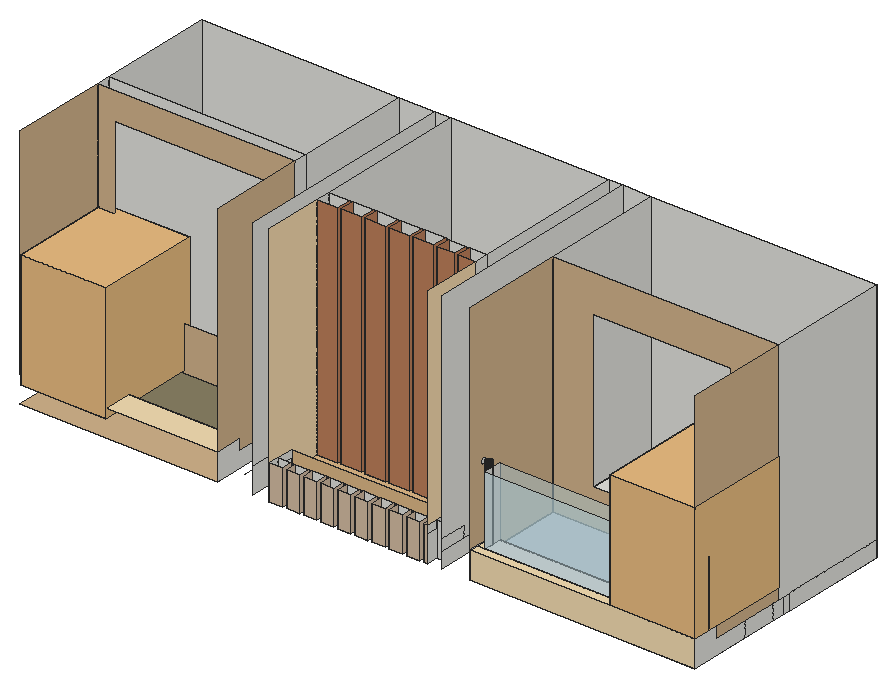
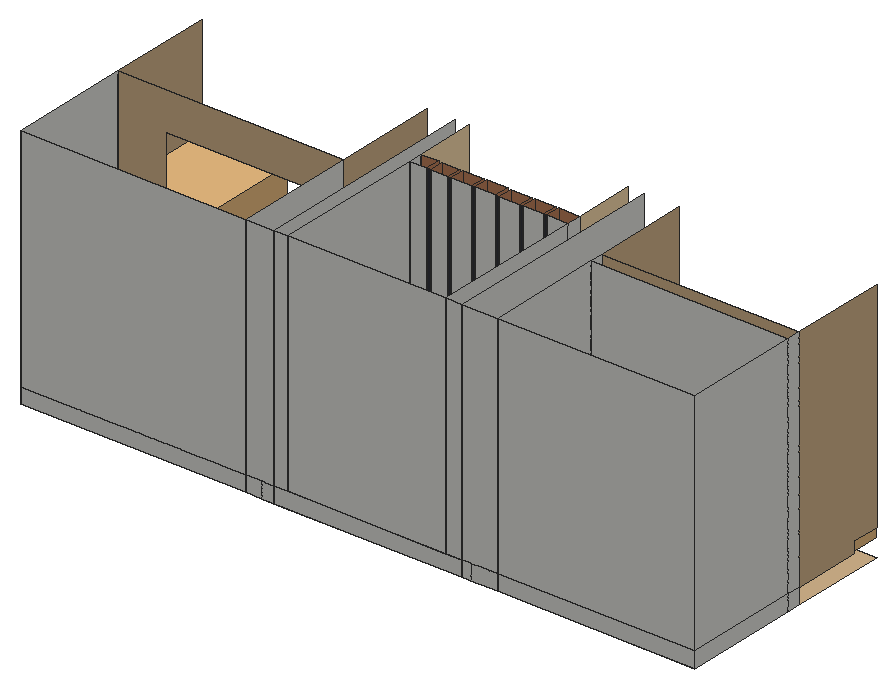
# SketchUp Ruby script. Lengths in inches.
U = 1.inch
M = Sketchup.active_model
def pt(a) = Geom::Point3d.new(a.map { |v| v * U })
def face(e, loops, mat)
  f = e.add_face(loops[0].map { |a| pt(a) })
  loops[1..].each { |l| e.add_face(l.map { |a| pt(a) }).erase! }
  f.material = f.back_material = mat if mat
  f
end
# faces: each face lists its corners as indices into pts; further lists are holes
def faces(e, pts, list, mat = nil) = list.each { |f| face(e, (f[0].is_a?(Array) ? f : [f]).map { |l| l.map { |i| pts[i] } }, mat) }
# xy, xz, yz: faces in a plane at the given z, y or x. An outline is a flat list of corners, or four numbers for a rectangle; further outlines are holes
def ring(l) = l.size == 4 ? [[l[0], l[1]], [l[2], l[1]], [l[2], l[3]], [l[0], l[3]]] : l.each_slice(2).to_a
def flat(e, list, mat, &to3) = list.each { |f| face(e, (f[0].is_a?(Array) ? f : [f]).map { |l| ring(l).map { |u, v| to3.(u, v) } }, mat) }
def xy(e, z, list, mat = nil) = flat(e, list, mat) { |x, y| [x, y, z] }
def xz(e, y, list, mat = nil) = flat(e, list, mat) { |x, z| [x, y, z] }
def yz(e, x, list, mat = nil) = flat(e, list, mat) { |y, z| [x, y, z] }
def lines(e, pts, list) = list.each { |a, b| e.add_line(pt(pts[a]), pt(pts[b])) }
# prism: a flat outline (further loops are holes) pulled along v
def prism(e, loops, v, mat = nil)
  f = face(e, loops, mat); d = Geom::Vector3d.new(v.map { |x| x * U })
  f.pushpull(f.normal.samedirection?(d) ? d.length : -d.length)
end
def box(e, o, s, mat = nil) = prism(e, [[o, [o[0] + s[0], o[1], o[2]], [o[0] + s[0], o[1] + s[1], o[2]], [o[0], o[1] + s[1], o[2]]]], [0, 0, s[2]], mat)
def at(x, y, z, deg = 0) = Geom::Transformation.translation(pt([x, y, z])) * Geom::Transformation.rotation(ORIGIN, Z_AXIS, deg.degrees)
def axes(o, x, y, z) = Geom::Transformation.new([*x, 0, *y, 0, *z, 0, *pt(o).to_a, 1])
def part(name) = M.definitions.add(name)
# library, detail: a bought-in or finely detailed component or shape, given as its bounding box
def library(name, o, s) = part(name).tap { |d| box(d.entities, o, s) }
def detail(e, o, s) = box(e.add_group.entities, o, s)
def put(e, d, t, mat = nil) = e.add_instance(d, t).tap { |i| i.material = mat if mat }
def group(e, t, mat = nil) = e.add_group.tap { |g| g.transformation = t; g.material = mat if mat }.entities
root = M.entities
M.materials.add("[0027_PeachPuff]").color = [255, 218, 185]
M.materials.add("[0034_Wheat]").color = [245, 222, 179]
M.materials.add("[0035_Tan]").color = [210, 180, 140]
M.materials.add("[0036_BurlyWood]1").color = [222, 184, 135]
M.materials.add("[Carpet Pattern Squares Multi]").color = [138, 129, 101]
M.materials.add("[Formica Beige]").color = [247, 219, 174]
M.materials.add("[Formica Laminate Dark]").color = [50, 53, 60]
M.materials.add("[Formica Laminate Light]").color = [213, 189, 164]
M.materials.add("[Marble Carrara Floor Tile]").color = [204, 208, 219]
M.materials.add("[Translucent Glass Safety]").color = [204, 235, 244]
M.materials["[Translucent Glass Safety]"].alpha = 0.5
M.materials.add("[Wood Veneer 02]").color = [190, 128, 91]
c1 = library("chau cay",[-24.34,-109.24,0],[56.46,62.58,79.69])
xy(root,1615.875,[[800.41,433.79,848.4,457.98],[856.53,433.79,904.52,457.98],[912.66,433.79,960.65,457.98],[968.78,433.79,1016.77,457.98],[1024.91,433.79,1072.9,457.98],
  [1081.03,433.79,1129.02,457.98],[1137.16,433.79,1185.15,457.98],[1192.22,433.79,1232.95,457.98],[1240.21,433.79,1272.8,457.98],[58.44,584.29,646.67,623.89],
  [646.67,584.29,752.97,623.89],[752.97,584.29,1313.62,623.89],[1313.62,584.29,1398.32,623.89],[58.44,623.89,646.67,971.67],[646.67,623.89,752.97,971.67],
  [752.97,623.89,1313.62,971.67],[1313.62,623.89,1398.32,971.67],[1398.32,647.48,2069.85,971.67]])
xy(root,1615.875,[[800.41,328.44,800.41,433.79,848.4,433.79,848.4,457.98,856.53,457.98,856.53,433.79,904.52,433.79,904.52,457.98,912.66,457.98,912.66,433.79,960.65,433.79,960.65,457.98,968.78,457.98,968.78,433.79,1016.77,433.79,1016.77,457.98,1024.91,457.98,1024.91,433.79,1072.9,433.79,1072.9,457.98,1081.03,457.98,1081.03,433.79,1129.02,433.79,1129.02,457.98,1137.16,457.98,1137.16,433.79,1185.15,433.79,1185.15,457.98,1192.22,457.98,1192.22,433.79,1232.95,433.79,1232.95,457.98,1240.21,457.98,1240.21,433.79,1272.8,433.79,1272.8,328.44]],"[0027_PeachPuff]")
xy(root,1615.875,[[58.44,295.82,646.67,584.29],[1398.32,295.82,2069.85,584.29],[1398.32,584.29,2069.85,623.89],[1398.32,623.89,2069.85,647.48]],"[0035_Tan]")
xy(root,1615.875,[[800.41,295.82,840.05,328.44],[851.53,295.82,891.17,328.44],[902.66,295.82,942.3,328.44],[953.78,295.82,993.42,328.44],[1004.91,295.82,1044.55,328.44],
  [1056.03,295.82,1095.67,328.44],[1107.16,295.82,1146.8,328.44],[1158.28,295.82,1197.92,328.44],[1209.41,295.82,1249.05,328.44],[1260.53,295.82,1272.8,328.44]],"[Formica Laminate Light]")
xy(root,1662.5625,[[752.97,378.54,800.41,971.67],[1272.8,378.54,1313.62,971.67],[800.41,474.79,862.92,517.1],[871.91,474.79,934.42,517.1],[943.41,474.79,1005.92,517.1],
  [1014.91,474.79,1077.42,517.1],[1086.41,474.79,1148.92,517.1],[1157.91,474.79,1210.375,517.1],[1220.42,474.79,1272.8,517.1],[800.41,517.1,1272.8,971.67],
  [58.44,584.29,646.67,623.89],[1398.32,606.67,2069.85,971.67],[58.44,623.89,646.67,971.67]])
xy(root,1662.5625,[[800.41,378.54,1272.8,378.54,1272.8,474.79,1220.42,474.79,1220.42,517.1,1210.375,517.1,1210.375,474.79,1157.91,474.79,1157.91,517.1,1148.92,517.1,1148.92,474.79,1086.41,474.79,1086.41,517.1,1077.42,517.1,1077.42,474.79,1014.91,474.79,1014.91,517.1,1005.92,517.1,1005.92,474.79,943.41,474.79,943.41,517.1,934.42,517.1,934.42,474.79,871.91,474.79,871.91,517.1,862.92,517.1,862.92,474.79,800.41,474.79]],"[0036_BurlyWood]1")
xy(root,1662.5625,[[58.44,378.54,646.67,584.29]],"[Carpet Pattern Squares Multi]")
xy(root,1662.5625,[[1398.32,378.54,2069.85,606.67]],"[Marble Carrara Floor Tile]")
xy(root,1695.75,[[1423.33,322.36,2046.06,378.54],[1413.02,338.97,1411.98,339.01,1410.95,339.17,1409.95,339.43,1408.97,339.8,1408.04,340.27,1407.17,340.83,1406.36,341.48,1405.62,342.21,1404.96,343.02,1404.39,343.89,1403.91,344.81,1403.53,345.78,1403.26,346.78,1403.09,347.81,1403.03,348.85,1403.08,349.89,1403.23,350.91,1403.5,351.92,1403.86,352.89,1404.33,353.82,1404.89,354.7,1405.54,355.51,1406.27,356.25,1407.08,356.91,1407.95,357.48,1408.87,357.96,1409.84,358.34,1410.84,358.61,1411.87,358.78,1412.91,358.84,1413.95,358.79,1414.97,358.64,1415.98,358.37,1416.95,358,1417.88,357.54,1418.76,356.98,1419.57,356.33,1420.3125,355.59,1420.97,354.79,1421.54,353.92,1422.02,353,1422.4,352.03,1422.67,351.02,1422.84,350,1422.9,348.96,1422.85,347.92,1422.7,346.89,1422.43,345.89,1422.07,344.91,1421.6,343.98,1421.04,343.11,1420.39,342.3,1419.66,341.56,1418.85,340.9,1417.98,340.33,1417.06,339.85,1416.09,339.47,1415.09,339.19,1414.06,339.03],[2056.33,338.97,2055.29,339.01,2054.27,339.17,2053.26,339.43,2052.29,339.8,2051.36,340.27,2050.48,340.83,2049.67,341.48,2048.93,342.21,2048.27,343.02,2047.7,343.89,2047.22,344.81,2046.84,345.78,2046.57,346.78,2046.4,347.81,2046.34,348.85,2046.39,349.89,2046.54,350.91,2046.81,351.92,2047.18,352.89,2047.64,353.82,2048.2,354.7,2048.85,355.51,2049.58,356.25,2050.39,356.91,2051.26,357.48,2052.18,357.96,2053.15,358.34,2054.15,358.61,2055.18,358.78,2056.22,358.84,2057.26,358.79,2058.29,358.64,2059.29,358.37,2060.27,358,2061.2,357.54,2062.07,356.98,2062.88,356.33,2063.625,355.59,2064.28,354.79,2064.85,353.92,2065.33,353,2065.71,352.03,2065.98,351.02,2066.15,350,2066.21,348.96,2066.17,347.92,2066.01,346.89,2065.75,345.89,2065.38,344.91,2064.91,343.98,2064.35,343.11,2063.7,342.3,2062.97,341.56,2062.16,340.9,2061.29,340.33,2060.37,339.85,2059.4,339.47,2058.4,339.19,2057.37,339.03]])
xy(root,1695.75,[[58.44,295.82,646.67,378.54],[1398.32,295.82,2069.85,322.36],[[1398.32,322.36,1423.33,378.54],[1413.02,338.97,1411.98,339.01,1410.95,339.17,1409.95,339.43,1408.97,339.8,1408.04,340.27,1407.17,340.83,1406.36,341.48,1405.62,342.21,1404.96,343.02,1404.39,343.89,1403.91,344.81,1403.53,345.78,1403.26,346.78,1403.09,347.81,1403.03,348.85,1403.08,349.89,1403.23,350.91,1403.5,351.92,1403.86,352.89,1404.33,353.82,1404.89,354.7,1405.54,355.51,1406.27,356.25,1407.08,356.91,1407.95,357.48,1408.87,357.96,1409.84,358.34,1410.84,358.61,1411.87,358.78,1412.91,358.84,1413.95,358.79,1414.97,358.64,1415.98,358.37,1416.95,358,1417.88,357.54,1418.76,356.98,1419.57,356.33,1420.3125,355.59,1420.97,354.79,1421.54,353.92,1422.02,353,1422.4,352.03,1422.67,351.02,1422.84,350,1422.9,348.96,1422.85,347.92,1422.7,346.89,1422.43,345.89,1422.07,344.91,1421.6,343.98,1421.04,343.11,1420.39,342.3,1419.66,341.56,1418.85,340.9,1417.98,340.33,1417.06,339.85,1416.09,339.47,1415.09,339.19,1414.06,339.03]],[[2046.06,322.36,2069.85,378.54],[2056.33,338.97,2055.29,339.01,2054.27,339.17,2053.26,339.43,2052.29,339.8,2051.36,340.27,2050.48,340.83,2049.67,341.48,2048.93,342.21,2048.27,343.02,2047.7,343.89,2047.22,344.81,2046.84,345.78,2046.57,346.78,2046.4,347.81,2046.34,348.85,2046.39,349.89,2046.54,350.91,2046.81,351.92,2047.18,352.89,2047.64,353.82,2048.2,354.7,2048.85,355.51,2049.58,356.25,2050.39,356.91,2051.26,357.48,2052.18,357.96,2053.15,358.34,2054.15,358.61,2055.18,358.78,2056.22,358.84,2057.26,358.79,2058.29,358.64,2059.29,358.37,2060.27,358,2061.2,357.54,2062.07,356.98,2062.88,356.33,2063.625,355.59,2064.28,354.79,2064.85,353.92,2065.33,353,2065.71,352.03,2065.98,351.02,2066.15,350,2066.21,348.96,2066.17,347.92,2066.01,346.89,2065.75,345.89,2065.38,344.91,2064.91,343.98,2064.35,343.11,2063.7,342.3,2062.97,341.56,2062.16,340.9,2061.29,340.33,2060.37,339.85,2059.4,339.47,2058.4,339.19,2057.37,339.03]]],"[0034_Wheat]")
xz(root,295.82,[[1398.32,1615.875,2069.85,1695.75]],"[0034_Wheat]")
xz(root,295.82,[[800.41,1615.875,840.05,1718.875],[851.53,1615.875,891.17,1718.875],[902.66,1615.875,942.3,1718.875],[953.78,1615.875,993.42,1718.875],[1004.91,1615.875,1044.55,1718.875],
  [1056.03,1615.875,1095.67,1718.875],[1107.16,1615.875,1146.8,1718.875],[1158.28,1615.875,1197.92,1718.875],[1209.41,1615.875,1249.05,1718.875],[1260.53,1615.875,1272.8,1718.875]],"[Formica Laminate Light]")
xz(root,322.36,[[1423.33,1695.75,2046.06,1901.1875]],"[Translucent Glass Safety]")
xz(root,328.44,[[800.41,1615.875,840.05,1718.875],[851.53,1615.875,891.17,1718.875],[902.66,1615.875,942.3,1718.875],[953.78,1615.875,993.42,1718.875],[1004.91,1615.875,1044.55,1718.875],
  [1056.03,1615.875,1095.67,1718.875],[1107.16,1615.875,1146.8,1718.875],[1158.28,1615.875,1197.92,1718.875],[1209.41,1615.875,1249.05,1718.875],[1260.53,1615.875,1272.8,1718.875],
  [1272.8,1615.875,1300.17,1718.875]])
xz(root,328.44,[[840.05,1615.875,851.53,1718.875],[891.17,1615.875,902.66,1718.875],[942.3,1615.875,953.78,1718.875],[993.42,1615.875,1004.91,1718.875],[1044.55,1615.875,1056.03,1718.875],
  [1095.67,1615.875,1107.16,1718.875],[1146.8,1615.875,1158.28,1718.875],[1197.92,1615.875,1209.41,1718.875],[1249.05,1615.875,1260.53,1718.875]],"[Formica Laminate Dark]")
xz(root,378.54,[[752.97,1662.5625,800.41,1695.75],[1272.8,1662.5625,1313.62,1695.75],[1398.32,1662.5625,2069.85,1695.75]])
xz(root,378.54,[[58.44,1662.5625,646.67,1695.75]],"[0034_Wheat]")
xz(root,378.54,[[800.41,1662.5625,1272.8,1718.875]],"[0036_BurlyWood]1")
xz(root,378.54,[[1423.33,1695.75,2046.06,1901.1875]],"[Translucent Glass Safety]")
xz(root,474.79,[[800.41,1662.5625,862.92,2344.3125],[871.91,1662.5625,934.42,2344.3125],[943.41,1662.5625,1005.92,2344.3125],[1014.91,1662.5625,1077.42,2344.3125],[1086.41,1662.5625,1148.92,2344.3125],
  [1157.91,1662.5625,1210.375,2344.3125],[1220.42,1662.5625,1272.8,2344.3125]],"[Wood Veneer 02]")
xz(root,517.1,[[800.41,1662.5625,862.92,2344.3125],[871.91,1662.5625,934.42,2344.3125],[943.41,1662.5625,1005.92,2344.3125],[1014.91,1662.5625,1077.42,2344.3125],[1086.41,1662.5625,1148.92,2344.3125],
  [1157.91,1662.5625,1210.375,2344.3125],[1220.42,1662.5625,1272.8,2344.3125]])
xz(root,517.1,[[862.92,1662.5625,871.91,2344.3125],[934.42,1662.5625,943.41,2344.3125],[1005.92,1662.5625,1014.91,2344.3125],[1077.42,1662.5625,1086.41,2344.3125],[1148.92,1662.5625,1157.91,2344.3125],
  [1210.375,1662.5625,1220.42,2344.3125]],"[Formica Laminate Dark]")
xz(root,584.29,[[[58.44,1662.5625,646.67,2344.3125],[108.51,1794.2,576.32,2262.01]]],"[0035_Tan]")
xz(root,606.67,[[[1398.32,1662.5625,2069.85,2344.3125],[1516.53,1770.73,1927.28,2231.42]]],"[0035_Tan]")
xz(root,623.89,[[58.44,1662.5625,646.67,2344.3125]])
xz(root,971.67,[[58.44,1615.875,646.67,1662.5625],[646.67,1615.875,726.78,1662.5625],[726.78,1615.875,752.97,1662.5625],[752.97,1615.875,1313.62,1662.5625],[1313.62,1615.875,1351.23,1662.5625],
  [1351.23,1615.875,1398.32,1662.5625],[1398.32,1615.875,2069.85,1662.5625],[58.44,1662.5625,646.67,2344.3125],[646.67,1662.5625,752.97,2344.3125],[752.97,1662.5625,800.41,2344.3125],
  [800.41,1662.5625,1272.8,2344.3125],[1272.8,1662.5625,1313.62,2344.3125],[1313.62,1662.5625,1398.32,2344.3125],[1398.32,1662.5625,2069.85,2344.3125]])
yz(root,58.44,[[584.29,1615.875,623.89,1662.5625],[623.89,1615.875,971.67,1662.5625],[584.29,1662.5625,623.89,2344.3125],[623.89,1662.5625,971.67,2344.3125]])
yz(root,58.44,[[378.54,1662.5625,584.29,1662.5625,584.29,2344.3125,295.82,2344.3125,295.82,1695.75,378.54,1695.75]],"[0035_Tan]")
yz(root,646.67,[[295.82,1615.875,295.82,1695.75,378.54,1695.75,378.54,1662.5625,971.67,1662.5625,971.67,1615.875],[584.29,1662.5625,623.89,2344.3125],[623.89,1662.5625,971.67,2344.3125]])
yz(root,646.67,[[378.54,1662.5625,378.54,1695.75,295.82,1695.75,295.82,2344.3125,584.29,2344.3125,584.29,1662.5625]],"[0035_Tan]")
yz(root,752.97,[[295.82,1615.875,295.82,1695.75,378.54,1695.75,378.54,1662.5625,971.67,1662.5625,971.67,1615.875],[378.54,1662.5625,378.54,1695.75,295.82,1695.75,295.82,2344.3125,971.67,2344.3125,971.67,1662.5625]])
yz(root,800.41,[[295.82,1615.875,328.44,1695.75],[474.79,1662.5625,517.1,2344.3125],[517.1,1662.5625,971.67,2344.3125],[295.82,1695.75,328.44,1718.875],[328.44,1695.75,378.54,1718.875]])
yz(root,800.41,[[378.54,1662.5625,474.79,1662.5625,474.79,2344.3125,295.82,2344.3125,295.82,1718.875,378.54,1718.875]],"[Formica Beige]")
yz(root,840.05,[[295.82,1615.875,328.44,1718.875]],"[Formica Laminate Light]")
yz(root,851.53,[[295.82,1615.875,328.44,1695.75],[295.82,1695.75,328.44,1718.875]],"[Formica Laminate Light]")
yz(root,862.92,[[474.79,1662.5625,517.1,2344.3125]],"[Wood Veneer 02]")
yz(root,871.91,[[474.79,1662.5625,517.1,2344.3125]],"[Wood Veneer 02]")
yz(root,891.17,[[295.82,1615.875,328.44,1718.875]],"[Formica Laminate Light]")
yz(root,902.66,[[295.82,1615.875,328.44,1695.75],[295.82,1695.75,328.44,1718.875]],"[Formica Laminate Light]")
yz(root,934.42,[[474.79,1662.5625,517.1,2344.3125]],"[Wood Veneer 02]")
yz(root,942.3,[[295.82,1615.875,328.44,1718.875]],"[Formica Laminate Light]")
yz(root,943.41,[[474.79,1662.5625,517.1,2344.3125]],"[Wood Veneer 02]")
yz(root,953.78,[[295.82,1615.875,328.44,1695.75],[295.82,1695.75,328.44,1718.875]],"[Formica Laminate Light]")
yz(root,993.42,[[295.82,1615.875,328.44,1718.875]],"[Formica Laminate Light]")
yz(root,1004.91,[[295.82,1615.875,328.44,1695.75],[295.82,1695.75,328.44,1718.875]],"[Formica Laminate Light]")
yz(root,1005.92,[[474.79,1662.5625,517.1,2344.3125]],"[Wood Veneer 02]")
yz(root,1014.91,[[474.79,1662.5625,517.1,2344.3125]],"[Wood Veneer 02]")
yz(root,1044.55,[[295.82,1615.875,328.44,1718.875]],"[Formica Laminate Light]")
yz(root,1056.03,[[295.82,1615.875,328.44,1695.75],[295.82,1695.75,328.44,1718.875]],"[Formica Laminate Light]")
yz(root,1077.42,[[474.79,1662.5625,517.1,2344.3125]],"[Wood Veneer 02]")
yz(root,1086.41,[[474.79,1662.5625,517.1,2344.3125]],"[Wood Veneer 02]")
yz(root,1095.67,[[295.82,1615.875,328.44,1718.875]],"[Formica Laminate Light]")
yz(root,1107.16,[[295.82,1615.875,328.44,1695.75],[295.82,1695.75,328.44,1718.875]],"[Formica Laminate Light]")
yz(root,1146.8,[[295.82,1615.875,328.44,1718.875]],"[Formica Laminate Light]")
yz(root,1148.92,[[474.79,1662.5625,517.1,2344.3125]],"[Wood Veneer 02]")
yz(root,1157.91,[[474.79,1662.5625,517.1,2344.3125]],"[Wood Veneer 02]")
yz(root,1158.28,[[295.82,1615.875,328.44,1695.75],[295.82,1695.75,328.44,1718.875]],"[Formica Laminate Light]")
yz(root,1197.92,[[295.82,1615.875,328.44,1718.875]],"[Formica Laminate Light]")
yz(root,1209.41,[[295.82,1615.875,328.44,1695.75],[295.82,1695.75,328.44,1718.875]],"[Formica Laminate Light]")
yz(root,1210.375,[[474.79,1662.5625,517.1,2344.3125]],"[Wood Veneer 02]")
yz(root,1220.42,[[474.79,1662.5625,517.1,2344.3125]],"[Wood Veneer 02]")
yz(root,1249.05,[[295.82,1615.875,328.44,1718.875]],"[Formica Laminate Light]")
yz(root,1260.53,[[295.82,1615.875,328.44,1695.75],[295.82,1695.75,328.44,1718.875]],"[Formica Laminate Light]")
yz(root,1272.8,[[295.82,1615.875,328.44,1695.75],[474.79,1662.5625,517.1,2344.3125],[517.1,1662.5625,971.67,2344.3125],[295.82,1695.75,328.44,1718.875],[328.44,1695.75,378.54,1718.875]])
yz(root,1272.8,[[378.54,1662.5625,378.54,1718.875,295.82,1718.875,295.82,2344.3125,474.79,2344.3125,474.79,1662.5625]],"[Formica Beige]")
yz(root,1313.62,[[295.82,1615.875,971.67,1662.5625],[295.82,1662.5625,378.54,1695.75],[378.54,1662.5625,971.67,1662.5625,971.67,2344.3125,295.82,2344.3125,295.82,1695.75,378.54,1695.75]])
yz(root,1398.32,[[295.82,1615.875,971.67,1662.5625],[295.82,1662.5625,378.54,1695.75],[606.67,1662.5625,971.67,2344.3125]])
yz(root,1398.32,[[[378.54,1662.5625,606.67,1662.5625,606.67,2344.3125,295.82,2344.3125,295.82,1695.75,378.54,1695.75],[347.7,1902.74,346.67,1902.8,345.64,1902.97,344.64,1903.24,343.67,1903.62,342.74,1904.1,341.875,1904.67,341.07,1905.33,340.34,1906.07,339.6875,1906.88,339.13,1907.76,338.66,1908.6875,338.29,1909.66,338.03,1910.67,337.87,1911.7,337.82,1912.73,337.88,1913.77,338.05,1914.8,338.33,1915.8,338.71,1916.77,339.18,1917.7,339.76,1918.56,340.41,1919.37,341.15,1920.1,341.97,1920.75,342.84,1921.3125,343.77,1921.78,344.75,1922.15,345.75,1922.41,346.78,1922.57,347.82,1922.62,348.86,1922.55,349.88,1922.39,350.89,1922.11,351.86,1921.73,352.78,1921.26,353.65,1920.68,354.45,1920.02,355.18,1919.28,355.83,1918.47,356.4,1917.6,356.86,1916.67,357.23,1915.69,357.49,1914.6875,357.65,1913.66,357.7,1912.62,357.64,1911.58,357.47,1910.56,357.2,1909.55,356.82,1908.58,356.34,1907.66,355.77,1906.79,355.11,1905.99,354.37,1905.25,353.56,1904.6,352.68,1904.04,351.75,1903.58,350.78,1903.21,349.77,1902.95,348.74,1902.79]]],"[0035_Tan]")
yz(root,1423.33,[[322.36,1695.75,378.54,1901.1875]])
yz(root,2046.06,[[322.36,1695.75,378.54,1901.1875]])
yz(root,2069.85,[[295.82,1615.875,481.57,1615.875,481.57,1662.5625,378.54,1662.5625,378.54,1695.75,295.82,1695.75],[481.57,1615.875,584.29,1662.5625],[584.29,1615.875,623.89,1662.5625],[623.89,1615.875,647.48,1662.5625],[647.48,1615.875,971.67,1662.5625],
  [606.67,1662.5625,971.67,2344.3125]])
yz(root,2069.85,[[[378.54,1662.5625,378.54,1695.75,295.82,1695.75,295.82,2344.3125,606.67,2344.3125,606.67,1662.5625],[347.7,1902.74,348.74,1902.79,349.77,1902.95,350.78,1903.21,351.75,1903.58,352.68,1904.04,353.56,1904.6,354.37,1905.25,355.11,1905.99,355.77,1906.79,356.34,1907.66,356.82,1908.58,357.2,1909.55,357.47,1910.56,357.64,1911.58,357.7,1912.62,357.65,1913.66,357.49,1914.6875,357.23,1915.69,356.86,1916.67,356.4,1917.6,355.83,1918.47,355.18,1919.28,354.45,1920.02,353.65,1920.68,352.78,1921.26,351.86,1921.73,350.89,1922.11,349.88,1922.39,348.86,1922.55,347.82,1922.62,346.78,1922.57,345.75,1922.41,344.75,1922.15,343.77,1921.78,342.84,1921.3125,341.97,1920.75,341.15,1920.1,340.41,1919.37,339.76,1918.56,339.18,1917.7,338.71,1916.77,338.33,1915.8,338.05,1914.8,337.88,1913.77,337.82,1912.73,337.87,1911.7,338.03,1910.67,338.29,1909.66,338.66,1908.6875,339.13,1907.76,339.6875,1906.88,340.34,1906.07,341.07,1905.33,341.875,1904.67,342.74,1904.1,343.67,1903.62,344.64,1903.24,345.64,1902.97,346.67,1902.8]]],"[0035_Tan]")
p = [[1410.95,339.17,1695.75],[1411.98,339.01,1695.75],[1411.98,339.01,1916.77],[1410.95,339.17,1916.77],[1413.02,338.97,1695.75],[1413.02,338.97,1916.77],
  [1414.06,339.03,1695.75],[1414.06,339.03,1916.77],[1415.09,339.19,1695.75],[1415.09,339.19,1916.77],[2054.27,339.17,1695.75],[2055.29,339.01,1695.75],
  [2055.29,339.01,1912.73],[2054.27,339.17,1912.73],[2056.33,338.97,1695.75],[2056.33,338.97,1912.73],[2057.37,339.03,1695.75],[2057.37,339.03,1912.73],
  [2058.4,339.19,1695.75],[2058.4,339.19,1912.73],[1409.95,339.43,1695.75],[1409.95,339.43,1916.77],[1416.09,339.47,1695.75],[1416.09,339.47,1916.77],
  [2053.26,339.43,1695.75],[2053.26,339.43,1912.73],[2059.4,339.47,1695.75],[2059.4,339.47,1912.73],[1408.97,339.8,1695.75],[1408.97,339.8,1916.77],
  [2052.29,339.8,1695.75],[2052.29,339.8,1912.73],[1417.06,339.85,1695.75],[1417.06,339.85,1916.77],[2060.37,339.85,1695.75],[2060.37,339.85,1912.73],
  [1408.04,340.27,1695.75],[1408.04,340.27,1916.77],[1417.98,340.33,1695.75],[1417.98,340.33,1916.77],[2051.36,340.27,1695.75],[2051.36,340.27,1912.73],
  [2061.29,340.33,1695.75],[2061.29,340.33,1912.73],[1407.17,340.83,1695.75],[1407.17,340.83,1916.77],[1418.85,340.9,1695.75],[1418.85,340.9,1916.77],
  [2050.48,340.83,1695.75],[2050.48,340.83,1912.73],[2062.16,340.9,1695.75],[2062.16,340.9,1912.73],[1406.36,341.48,1695.75],[1406.36,341.48,1916.77],
  [2049.67,341.48,1695.75],[2049.67,341.48,1912.73],[1419.66,341.56,1695.75],[1419.66,341.56,1916.77],[2062.97,341.56,1695.75],[2062.97,341.56,1912.73],
  [1405.62,342.21,1695.75],[1405.62,342.21,1916.77],[2048.93,342.21,1695.75],[2048.93,342.21,1912.73],[1420.39,342.3,1695.75],[1420.39,342.3,1916.77],
  [2063.7,342.3,1695.75],[2063.7,342.3,1912.73],[1404.96,343.02,1695.75],[1404.96,343.02,1916.77],[2048.27,343.02,1695.75],[2048.27,343.02,1912.73],
  [1421.04,343.11,1695.75],[1421.04,343.11,1916.77],[2064.35,343.11,1695.75],[2064.35,343.11,1912.73],[1404.39,343.89,1695.75],[1404.39,343.89,1916.77],
  [2047.7,343.89,1695.75],[2047.7,343.89,1912.73],[1421.6,343.98,1695.75],[1421.6,343.98,1916.77],[2064.91,343.98,1695.75],[2064.91,343.98,1912.73],
  [1403.91,344.81,1695.75],[1403.91,344.81,1916.77],[2047.22,344.81,1695.75],[2047.22,344.81,1912.73],[1422.07,344.91,1695.75],[1422.07,344.91,1916.77],
  [2065.38,344.91,1695.75],[2065.38,344.91,1912.73],[1403.53,345.78,1695.75],[1403.53,345.78,1916.77],[2046.84,345.78,1695.75],[2046.84,345.78,1912.73],
  [1422.43,345.89,1695.75],[1422.43,345.89,1916.77],[2065.75,345.89,1695.75],[2065.75,345.89,1912.73],[1403.26,346.78,1695.75],[1403.26,346.78,1916.77],
  [2046.57,346.78,1695.75],[2046.57,346.78,1912.73],[1422.7,346.89,1695.75],[1422.7,346.89,1916.77],[2066.01,346.89,1695.75],[2066.01,346.89,1912.73],
  [1403.09,347.81,1695.75],[1403.09,347.81,1916.77],[2046.4,347.81,1695.75],[2046.4,347.81,1912.73],[1422.85,347.92,1695.75],[1422.85,347.92,1916.77],
  [2066.17,347.92,1695.75],[2066.17,347.92,1912.73],[1403.03,348.85,1695.75],[1403.03,348.85,1916.77],[2046.34,348.85,1695.75],[2046.34,348.85,1912.73],
  [1422.9,348.96,1695.75],[1422.9,348.96,1916.77],[2066.21,348.96,1695.75],[2066.21,348.96,1912.73],[1403.08,349.89,1695.75],[1403.08,349.89,1916.77],
  [2046.39,349.89,1695.75],[2046.39,349.89,1912.73],[1422.84,350,1695.75],[1422.84,350,1916.77],[2066.15,350,1695.75],[2066.15,350,1912.73],
  [1403.23,350.91,1695.75],[1403.23,350.91,1916.77],[2046.54,350.91,1695.75],[2046.54,350.91,1912.73],[1422.67,351.02,1695.75],[1422.67,351.02,1916.77],
  [2065.98,351.02,1695.75],[2065.98,351.02,1912.73],[1403.5,351.92,1695.75],[1403.5,351.92,1916.77],[2046.81,351.92,1695.75],[2046.81,351.92,1912.73],
  [1422.4,352.03,1695.75],[1422.4,352.03,1916.77],[2065.71,352.03,1695.75],[2065.71,352.03,1912.73],[1403.86,352.89,1695.75],[1403.86,352.89,1916.77],
  [2047.18,352.89,1695.75],[2047.18,352.89,1912.73],[1422.02,353,1695.75],[1422.02,353,1916.77],[2065.33,353,1695.75],[2065.33,353,1912.73],
  [1404.33,353.82,1695.75],[1404.33,353.82,1916.77],[2047.64,353.82,1695.75],[2047.64,353.82,1912.73],[1421.54,353.92,1695.75],[1421.54,353.92,1916.77],
  [2064.85,353.92,1695.75],[2064.85,353.92,1912.73],[1404.89,354.7,1695.75],[1404.89,354.7,1916.77],[2048.2,354.7,1695.75],[2048.2,354.7,1912.73],
  [1420.97,354.79,1695.75],[1420.97,354.79,1916.77],[2064.28,354.79,1695.75],[2064.28,354.79,1912.73],[1405.54,355.51,1695.75],[1405.54,355.51,1916.77],
  [2048.85,355.51,1695.75],[2048.85,355.51,1912.73],[1420.3125,355.59,1695.75],[1420.3125,355.59,1916.77],[2063.625,355.59,1695.75],[2063.625,355.59,1912.73],
  [1406.27,356.25,1695.75],[1406.27,356.25,1916.77],[2049.58,356.25,1695.75],[2049.58,356.25,1912.73],[1419.57,356.33,1695.75],[1419.57,356.33,1916.77],
  [2062.88,356.33,1695.75],[2062.88,356.33,1912.73],[1407.08,356.91,1695.75],[1407.08,356.91,1916.77],[2050.39,356.91,1695.75],[2050.39,356.91,1912.73],
  [1418.76,356.98,1695.75],[1418.76,356.98,1916.77],[2062.07,356.98,1695.75],[2062.07,356.98,1912.73],[1407.95,357.48,1695.75],[1407.95,357.48,1916.77],
  [2051.26,357.48,1695.75],[2051.26,357.48,1912.73],[1417.88,357.54,1695.75],[1417.88,357.54,1916.77],[2061.2,357.54,1695.75],[2061.2,357.54,1912.73],
  [1408.87,357.96,1695.75],[1408.87,357.96,1916.77],[1416.95,358,1695.75],[1416.95,358,1916.77],[2052.18,357.96,1695.75],[2052.18,357.96,1912.73],
  [2060.27,358,1695.75],[2060.27,358,1912.73],[1409.84,358.34,1695.75],[1409.84,358.34,1916.77],[1415.98,358.37,1695.75],[1415.98,358.37,1916.77],
  [2053.15,358.34,1695.75],[2053.15,358.34,1912.73],[2059.29,358.37,1695.75],[2059.29,358.37,1912.73],[1410.84,358.61,1695.75],[1410.84,358.61,1916.77],
  [2054.15,358.61,1695.75],[2054.15,358.61,1912.73],[1414.97,358.64,1695.75],[1414.97,358.64,1916.77],[2058.29,358.64,1695.75],[2058.29,358.64,1912.73],
  [1411.87,358.78,1695.75],[1411.87,358.78,1916.77],[1413.95,358.79,1695.75],[1413.95,358.79,1916.77],[2055.18,358.78,1695.75],[2055.18,358.78,1912.73],
  [2057.26,358.79,1695.75],[2057.26,358.79,1912.73],[1412.91,358.84,1695.75],[1412.91,358.84,1916.77],[2056.22,358.84,1695.75],[2056.22,358.84,1912.73],
  [726.78,971.67,1662.5625],[726.78,295.82,1662.5625]]
faces(root,p,[[0,1,2,3],[1,4,5,2],[4,6,7,5],[6,8,9,7],[10,11,12,13],[11,14,15,12],[14,16,17,15],[16,18,19,17],
  [20,0,3,21],[8,22,23,9],[24,10,13,25],[18,26,27,19],[28,20,21,29],[30,24,25,31],[22,32,33,23],[26,34,35,27],
  [36,28,29,37],[32,38,39,33],[40,30,31,41],[34,42,43,35],[44,36,37,45],[38,46,47,39],[48,40,41,49],[42,50,51,43],
  [52,44,45,53],[54,48,49,55],[46,56,57,47],[50,58,59,51],[60,52,53,61],[62,54,55,63],[56,64,65,57],[58,66,67,59],
  [68,60,61,69],[70,62,63,71],[64,72,73,65],[66,74,75,67],[76,68,69,77],[78,70,71,79],[72,80,81,73],[74,82,83,75],
  [84,76,77,85],[86,78,79,87],[80,88,89,81],[82,90,91,83],[92,84,85,93],[94,86,87,95],[88,96,97,89],[90,98,99,91],
  [100,92,93,101],[102,94,95,103],[96,104,105,97],[98,106,107,99],[108,100,101,109],[110,102,103,111],[104,112,113,105],[106,114,115,107],
  [116,108,109,117],[118,110,111,119],[112,120,121,113],[114,122,123,115],[124,116,117,125],[126,118,119,127],[120,128,129,121],[122,130,131,123],
  [132,124,125,133],[134,126,127,135],[128,136,137,129],[130,138,139,131],[140,132,133,141],[142,134,135,143],[136,144,145,137],[138,146,147,139],
  [148,140,141,149],[150,142,143,151],[144,152,153,145],[146,154,155,147],[156,148,149,157],[158,150,151,159],[152,160,161,153],[154,162,163,155],
  [164,156,157,165],[166,158,159,167],[160,168,169,161],[162,170,171,163],[172,164,165,173],[174,166,167,175],[168,176,177,169],[170,178,179,171],
  [180,172,173,181],[182,174,175,183],[176,184,185,177],[178,186,187,179],[188,180,181,189],[190,182,183,191],[184,192,193,185],[186,194,195,187],
  [196,188,189,197],[198,190,191,199],[192,200,201,193],[194,202,203,195],[204,196,197,205],[200,206,207,201],[208,198,199,209],[202,210,211,203],
  [212,204,205,213],[206,214,215,207],[216,208,209,217],[210,218,219,211],[220,212,213,221],[222,216,217,223],[214,224,225,215],[218,226,227,219],
  [228,220,221,229],[224,230,231,225],[232,222,223,233],[226,234,235,227],[236,228,229,237],[230,236,237,231],[238,232,233,239],[234,238,239,235]],"[Formica Laminate Dark]")
lines(root,p,[[240,241]])
put(root,c1,axes([169.76,64.16,1667.3125],[4.5,0,0],[0,-4.9651,0],[0,0,4.37432]))
put(root,c1,axes([1925.3125,64.16,1695.75],[4.5,0,0],[0,-4.9651,0],[0,0,4.37432]))
